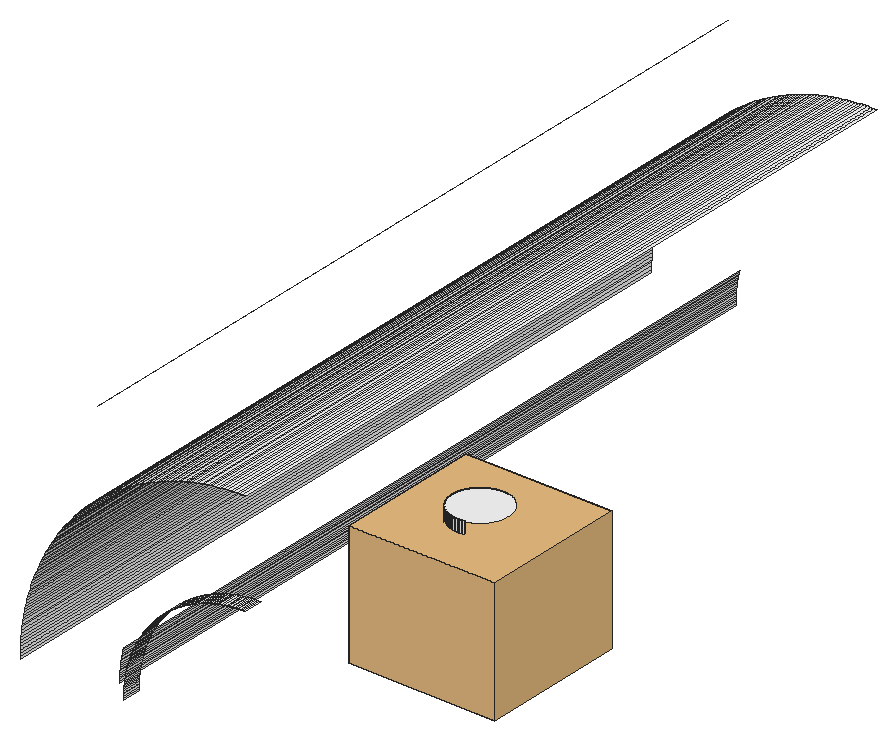
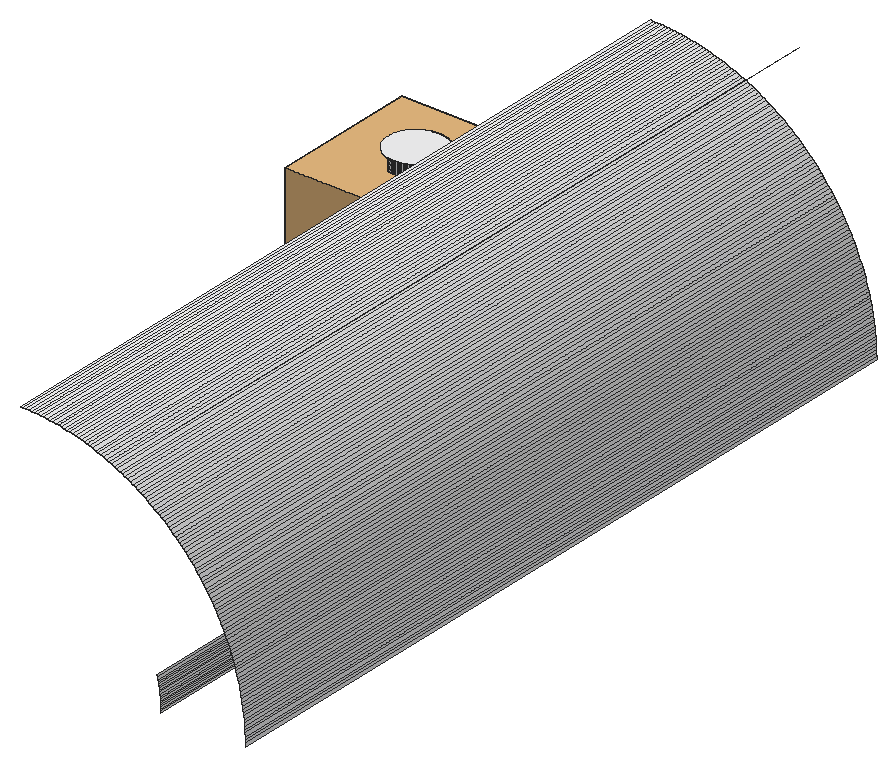
# SketchUp Ruby script. Lengths in inches.
U = 1.inch
M = Sketchup.active_model
def pt(a) = Geom::Point3d.new(a.map { |v| v * U })
def face(e, loops, mat)
  f = e.add_face(loops[0].map { |a| pt(a) })
  loops[1..].each { |l| e.add_face(l.map { |a| pt(a) }).erase! }
  f.material = f.back_material = mat if mat
  f
end
# faces: each face lists its corners as indices into pts; further lists are holes
def faces(e, pts, list, mat = nil) = list.each { |f| face(e, (f[0].is_a?(Array) ? f : [f]).map { |l| l.map { |i| pts[i] } }, mat) }
# xy, xz, yz: faces in a plane at the given z, y or x. An outline is a flat list of corners, or four numbers for a rectangle; further outlines are holes
def ring(l) = l.size == 4 ? [[l[0], l[1]], [l[2], l[1]], [l[2], l[3]], [l[0], l[3]]] : l.each_slice(2).to_a
def flat(e, list, mat, &to3) = list.each { |f| face(e, (f[0].is_a?(Array) ? f : [f]).map { |l| ring(l).map { |u, v| to3.(u, v) } }, mat) }
def xy(e, z, list, mat = nil) = flat(e, list, mat) { |x, y| [x, y, z] }
def xz(e, y, list, mat = nil) = flat(e, list, mat) { |x, z| [x, y, z] }
def yz(e, x, list, mat = nil) = flat(e, list, mat) { |y, z| [x, y, z] }
def lines(e, pts, list) = list.each { |a, b| e.add_line(pt(pts[a]), pt(pts[b])) }
# prism: a flat outline (further loops are holes) pulled along v
def prism(e, loops, v, mat = nil)
  f = face(e, loops, mat); d = Geom::Vector3d.new(v.map { |x| x * U })
  f.pushpull(f.normal.samedirection?(d) ? d.length : -d.length)
end
def box(e, o, s, mat = nil) = prism(e, [[o, [o[0] + s[0], o[1], o[2]], [o[0] + s[0], o[1] + s[1], o[2]], [o[0], o[1] + s[1], o[2]]]], [0, 0, s[2]], mat)
def at(x, y, z, deg = 0) = Geom::Transformation.translation(pt([x, y, z])) * Geom::Transformation.rotation(ORIGIN, Z_AXIS, deg.degrees)
def axes(o, x, y, z) = Geom::Transformation.new([*x, 0, *y, 0, *z, 0, *pt(o).to_a, 1])
def part(name) = M.definitions.add(name)
# library, detail: a bought-in or finely detailed component or shape, given as its bounding box
def library(name, o, s) = part(name).tap { |d| box(d.entities, o, s) }
def detail(e, o, s) = box(e.add_group.entities, o, s)
def put(e, d, t, mat = nil) = e.add_instance(d, t).tap { |i| i.material = mat if mat }
def group(e, t, mat = nil) = e.add_group.tap { |g| g.transformation = t; g.material = mat if mat }.entities
root = M.entities
M.materials.add("[Quartz Light Grey]").color = [251, 251, 252]
c1 = library("5",[-6.25,-6.25,-13.16],[15.58,15.58,13.16])
xy(root,115,[[59.66,187,59.83,189],[59.83,187,60,189]],"[Quartz Light Grey]")
xy(root,119.5,[[68.84,204,68.76,204.01,68.6875,204.02,68.61,204.03,68.45,204.05,68.375,204.07,68.3,204.08,68.22,204.1,68.15,204.125,68.07,204.15,68,204.17,67.92,204.2,67.71,204.29,67.64,204.33,67.57,204.36,67.43,204.44,67.37,204.48,67.3,204.53,67.24,204.57,67.17,204.62,66.93,204.82,66.88,204.88,66.82,204.93,66.62,205.17,66.57,205.24,66.53,205.3,66.48,205.37,66.44,205.43,66.36,205.57,66.33,205.64,66.29,205.71,66.2,205.92,66.17,206,66.15,206.07,66.125,206.15,66.1,206.22,66.08,206.3,66.07,206.375,66.05,206.45,66.03,206.61,66.02,206.6875,66.01,206.76,66,206.84,66,207.16,66.01,207.24,66.02,207.3125,66.03,207.39,66.05,207.55,66.07,207.625,66.08,207.7,66.1,207.78,66.125,207.85,66.15,207.93,66.17,208,66.2,208.08,66.29,208.29,66.33,208.36,66.36,208.43,66.44,208.57,66.48,208.63,66.53,208.7,66.57,208.76,66.62,208.83,66.82,209.07,66.88,209.12,66.93,209.18,67.17,209.38,67.24,209.43,67.3,209.47,67.37,209.52,67.43,209.56,67.57,209.64,67.64,209.67,67.71,209.71,67.92,209.8,68,209.83,68.07,209.85,68.15,209.875,68.22,209.9,68.3,209.92,68.375,209.93,68.45,209.95,68.61,209.97,68.6875,209.98,68.76,209.99,68.84,210,69.16,210,69.24,209.99,69.3125,209.98,69.39,209.97,69.55,209.95,69.625,209.93,69.7,209.92,69.78,209.9,69.85,209.875,69.93,209.85,70,209.83,70.08,209.8,70.29,209.71,70.36,209.67,70.43,209.64,70.57,209.56,70.63,209.52,70.7,209.47,70.76,209.43,70.83,209.38,71.07,209.18,71.12,209.12,71.18,209.07,71.38,208.83,71.43,208.76,71.47,208.7,71.52,208.63,71.56,208.57,71.64,208.43,71.67,208.36,71.71,208.29,71.8,208.08,71.83,208,71.85,207.93,71.875,207.85,71.9,207.78,71.92,207.7,71.93,207.625,71.95,207.55,71.97,207.39,71.98,207.3125,71.99,207.24,72,207.16,72,206.84,71.99,206.76,71.98,206.6875,71.97,206.61,71.95,206.45,71.93,206.375,71.92,206.3,71.9,206.22,71.875,206.15,71.85,206.07,71.83,206,71.8,205.92,71.71,205.71,71.67,205.64,71.64,205.57,71.56,205.43,71.52,205.37,71.47,205.3,71.43,205.24,71.38,205.17,71.18,204.93,71.12,204.88,71.07,204.82,70.83,204.62,70.76,204.57,70.7,204.53,70.63,204.48,70.57,204.44,70.43,204.36,70.36,204.33,70.29,204.29,70.08,204.2,70,204.17,69.93,204.15,69.85,204.125,69.78,204.1,69.7,204.08,69.625,204.07,69.55,204.05,69.39,204.03,69.3125,204.02,69.24,204.01,69.16,204]],"[Quartz Light Grey]")
xy(root,126,[[59.6875,187,60,271]],"[Quartz Light Grey]")
xz(root,204,[[68.84,117,68.92,119.5],[68.92,117,69,119.5],[69,117,69.08,119.5],[69.08,117,69.16,119.5]],"[Quartz Light Grey]")
xz(root,210,[[68.84,117,68.92,119.5],[68.92,117,69,119.5],[69,117,69.08,119.5],[69.08,117,69.16,119.5]],"[Quartz Light Grey]")
yz(root,36,[[187,102,271,102.3125]],"[Quartz Light Grey]")
yz(root,45,[[189,102,271,102.2]],"[Quartz Light Grey]")
yz(root,45.01,[[189,102.39,271,102.59]],"[Quartz Light Grey]")
yz(root,47,[[187,102,189,102.17],[187,102.17,189,102.34]],"[Quartz Light Grey]")
yz(root,66,[[206.84,117,206.92,119.5],[206.92,117,207,119.5],[207,117,207.08,119.5],[207.08,117,207.16,119.5]],"[Quartz Light Grey]")
p = [[45.01,271,102.39],[45.01,189,102.39],[45,189,102.2],[45,271,102.2],[36,187,102.3125],[36.01,187,102.63],
  [36.01,271,102.63],[36,271,102.3125],[47.01,187,102.51],[47,187,102.34],[47,189,102.34],[47.01,189,102.51],
  [47.02,187,102.68],[47.02,189,102.68],[36.02,187,102.94],[36.02,271,102.94],[45.02,271,102.79],[45.02,189,102.79],
  [45.01,189,102.59],[45.01,271,102.59],[47.03,187,102.85],[47.03,189,102.85],[45.03,271,102.98],[45.03,189,102.98],
  [36.03,187,103.26],[36.03,271,103.26],[47.04,187,103.02],[47.04,189,103.02],[47.05,187,103.19],[47.05,189,103.19],
  [45.05,271,103.18],[45.05,189,103.18],[47.07,187,103.36],[47.07,189,103.36],[45.0625,271,103.37],[45.0625,189,103.37],
  [36.05,187,103.57],[36.05,271,103.57],[47.09,187,103.53],[47.09,189,103.53],[45.08,271,103.57],[45.08,189,103.57],
  [47.11,187,103.7],[47.11,189,103.7],[36.07,187,103.88],[36.07,271,103.88],[45.1,271,103.76],[45.1,189,103.76],
  [47.13,187,103.87],[47.13,189,103.87],[45.13,271,103.96],[45.13,189,103.96],[36.1,187,104.2],[36.1,271,104.2],
  [47.16,187,104.03],[47.16,189,104.03],[47.1875,187,104.2],[47.1875,189,104.2],[45.16,271,104.15],[45.16,189,104.15],
  [36.13,187,104.51],[36.13,271,104.51],[47.22,187,104.37],[47.22,189,104.37],[45.18,271,104.35],[45.18,189,104.35],
  [45.22,271,104.54],[45.22,189,104.54],[47.25,187,104.54],[47.25,189,104.54],[36.17,187,104.82],[36.17,271,104.82],
  [47.28,187,104.7],[47.28,189,104.7],[45.25,271,104.73],[45.25,189,104.73],[47.32,187,104.87],[47.32,189,104.87],
  [45.29,271,104.93],[45.29,189,104.93],[36.21,187,105.13],[36.21,271,105.13],[47.36,187,105.03],[47.36,189,105.03],
  [45.33,271,105.12],[45.33,189,105.12],[47.4,187,105.2],[47.4,189,105.2],[36.25,187,105.44],[36.25,271,105.44],
  [45.37,271,105.31],[45.37,189,105.31],[47.44,187,105.36],[47.44,189,105.36],[45.41,271,105.5],[45.41,189,105.5],
  [36.3,187,105.75],[36.3,271,105.75],[47.49,187,105.53],[47.49,189,105.53],[47.54,187,105.69],[47.54,189,105.69],
  [47.58,187,105.86],[47.58,189,105.86],[36.35,187,106.0625],[36.35,271,106.0625],[47.64,187,106.02],[47.64,189,106.02],
  [47.69,187,106.18],[47.69,189,106.18],[36.4,187,106.375],[36.4,271,106.375],[47.75,187,106.34],[47.75,189,106.34],
  [47.8,187,106.5],[47.8,189,106.5],[36.46,187,106.68],[36.46,271,106.68],[47.86,187,106.66],[47.86,189,106.66],
  [36.52,187,106.99],[36.52,271,106.99],[47.93,187,106.82],[47.93,189,106.82],[47.99,187,106.97],[47.99,189,106.97],
  [36.59,187,107.3],[36.59,271,107.3],[48.06,187,107.13],[48.06,189,107.13],[48.125,187,107.29],[48.125,189,107.29],
  [36.66,187,107.6],[36.66,271,107.6],[48.19,187,107.44],[48.19,189,107.44],[48.27,187,107.6],[48.27,189,107.6],
  [36.74,187,107.91],[36.74,271,107.91],[48.34,187,107.75],[48.34,189,107.75],[48.42,187,107.9],[48.42,189,107.9],
  [36.82,187,108.21],[36.82,271,108.21],[48.5,187,108.05],[48.5,189,108.05],[48.58,187,108.2],[48.58,189,108.2],
  [36.9,187,108.51],[36.9,271,108.51],[48.66,187,108.35],[48.66,189,108.35],[48.74,187,108.5],[48.74,189,108.5],
  [36.99,187,108.82],[36.99,271,108.82],[48.83,187,108.65],[48.83,189,108.65],[48.92,187,108.79],[48.92,189,108.79],
  [37.08,187,109.12],[37.08,271,109.12],[49.01,187,108.9375],[49.01,189,108.9375],[49.1,187,109.08],[49.1,189,109.08],
  [37.17,187,109.42],[37.17,271,109.42],[49.19,187,109.22],[49.19,189,109.22],[49.29,187,109.36],[49.29,189,109.36],
  [37.27,187,109.71],[37.27,271,109.71],[49.38,187,109.5],[49.38,189,109.5],[49.48,187,109.64],[49.48,189,109.64],
  [49.58,187,109.78],[49.58,189,109.78],[37.375,187,110.01],[37.375,271,110.01],[49.6875,187,109.91],[49.6875,189,109.91],
  [49.79,187,110.05],[49.79,189,110.05],[37.48,187,110.31],[37.48,271,110.31],[49.9,187,110.18],[49.9,189,110.18],
  [50.01,187,110.3125],[50.01,189,110.3125],[37.59,187,110.6],[37.59,271,110.6],[50.11,187,110.44],[50.11,189,110.44],
  [50.23,187,110.57],[50.23,189,110.57],[37.71,187,110.89],[37.71,271,110.89],[50.34,187,110.7],[50.34,189,110.7],
  [50.45,187,110.82],[50.45,189,110.82],[50.57,187,110.95],[50.57,189,110.95],[37.83,187,111.18],[37.83,271,111.18],
  [50.6875,187,111.07],[50.6875,189,111.07],[50.81,187,111.19],[50.81,189,111.19],[37.95,187,111.47],[37.95,271,111.47],
  [50.93,187,111.3125],[50.93,189,111.3125],[51.05,187,111.43],[51.05,189,111.43],[51.18,187,111.55],[51.18,189,111.55],
  [38.07,187,111.76],[38.07,271,111.76],[51.3,187,111.66],[51.3,189,111.66],[51.43,187,111.77],[51.43,189,111.77],
  [38.2,187,112.05],[38.2,271,112.05],[51.56,187,111.89],[51.56,189,111.89],[51.6875,187,111.99],[51.6875,189,111.99],
  [38.34,187,112.33],[38.34,271,112.33],[51.82,187,112.1],[51.82,189,112.1],[51.95,187,112.21],[51.95,189,112.21],
  [52.09,187,112.3125],[52.09,189,112.3125],[38.48,187,112.61],[38.48,271,112.61],[52.22,187,112.42],[52.22,189,112.42],
  [52.36,187,112.52],[52.36,189,112.52],[52.5,187,112.62],[52.5,189,112.62],[38.62,187,112.9],[38.62,271,112.9],
  [52.64,187,112.71],[52.64,189,112.71],[52.78,187,112.81],[52.78,189,112.81],[52.92,187,112.9],[52.92,189,112.9],
  [38.76,187,113.17],[38.76,271,113.17],[53.0625,187,112.99],[53.0625,189,112.99],[53.21,187,113.08],[53.21,189,113.08],
  [53.35,187,113.17],[53.35,189,113.17],[38.91,187,113.45],[38.91,271,113.45],[53.5,187,113.26],[53.5,189,113.26],
  [53.65,187,113.34],[53.65,189,113.34],[53.8,187,113.42],[53.8,189,113.42],[53.95,187,113.5],[53.95,189,113.5],
  [39.06,187,113.73],[39.06,271,113.73],[54.1,187,113.58],[54.1,189,113.58],[54.25,187,113.66],[54.25,189,113.66],
  [39.22,187,114],[39.22,271,114],[54.4,187,113.73],[54.4,189,113.73],[54.56,187,113.81],[54.56,189,113.81],
  [54.71,187,113.875],[54.71,189,113.875],[54.87,187,113.94],[54.87,189,113.94],[55.03,187,114.01],[55.03,189,114.01],
  [39.375,187,114.27],[39.375,271,114.27],[55.18,187,114.07],[55.18,189,114.07],[55.34,187,114.14],[55.34,189,114.14],
  [55.5,187,114.2],[55.5,189,114.2],[55.66,187,114.25],[55.66,189,114.25],[39.54,187,114.54],[39.54,271,114.54],
  [55.82,187,114.31],[55.82,189,114.31],[55.98,187,114.36],[55.98,189,114.36],[56.14,187,114.42],[56.14,189,114.42],
  [56.31,187,114.46],[56.31,189,114.46],[39.7,187,114.81],[39.7,271,114.81],[56.47,187,114.51],[56.47,189,114.51],
  [56.64,187,114.56],[56.64,189,114.56],[56.8,187,114.6],[56.8,189,114.6],[56.97,187,114.64],[56.97,189,114.64],
  [57.13,187,114.68],[57.13,189,114.68],[57.3,187,114.72],[57.3,189,114.72],[57.46,187,114.75],[57.46,189,114.75],
  [39.87,187,115.07],[39.87,271,115.07],[57.63,187,114.78],[57.63,189,114.78],[57.8,187,114.8125],[57.8,189,114.8125],
  [57.97,187,114.84],[57.97,189,114.84],[58.13,187,114.87],[58.13,189,114.87],[58.3,187,114.89],[58.3,189,114.89],
  [58.47,187,114.91],[58.47,189,114.91],[58.64,187,114.93],[58.64,189,114.93],[58.81,187,114.95],[58.81,189,114.95],
  [58.98,187,114.96],[58.98,189,114.96],[59.15,187,114.97],[59.15,189,114.97],[59.32,187,114.98],[59.32,189,114.98],
  [59.49,187,114.99],[59.49,189,114.99],[59.66,187,115],[59.66,189,115],[40.04,187,115.33],[40.04,271,115.33],
  [40.22,187,115.59],[40.22,271,115.59],[40.4,187,115.85],[40.4,271,115.85],[40.58,187,116.11],[40.58,271,116.11],
  [40.77,187,116.36],[40.77,271,116.36],[40.96,187,116.61],[40.96,271,116.61],[41.15,187,116.86],[41.15,271,116.86],
  [41.35,187,117.1],[41.35,271,117.1],[68.53,204.04,117],[68.45,204.05,117],[68.45,204.05,119.5],[68.53,204.04,119.5],
  [68.61,204.03,117],[68.61,204.03,119.5],[68.6875,204.02,117],[68.6875,204.02,119.5],[68.76,204.01,117],[68.76,204.01,119.5],
  [68.84,204,117],[68.84,204,119.5],[69.24,204.01,117],[69.16,204,117],[69.16,204,119.5],[69.24,204.01,119.5],
  [69.3125,204.02,117],[69.3125,204.02,119.5],[69.39,204.03,117],[69.39,204.03,119.5],[69.47,204.04,117],[69.47,204.04,119.5],
  [69.55,204.05,117],[69.55,204.05,119.5],[68.07,204.15,117],[68,204.17,117],[68,204.17,119.5],[68.07,204.15,119.5],
  [68.15,204.125,117],[68.15,204.125,119.5],[68.22,204.1,117],[68.22,204.1,119.5],[68.3,204.08,117],[68.3,204.08,119.5],
  [68.375,204.07,117],[68.375,204.07,119.5],[69.625,204.07,117],[69.625,204.07,119.5],[69.7,204.08,117],[69.7,204.08,119.5],
  [67.85,204.23,117],[67.78,204.26,117],[67.78,204.26,119.5],[67.85,204.23,119.5],[67.92,204.2,117],[67.92,204.2,119.5],
  [67.64,204.33,117],[67.57,204.36,117],[67.57,204.36,119.5],[67.64,204.33,119.5],[67.71,204.29,117],[67.71,204.29,119.5],
  [67.43,204.44,117],[67.37,204.48,117],[67.37,204.48,119.5],[67.43,204.44,119.5],[67.5,204.4,117],[67.5,204.4,119.5],
  [67.3,204.53,117],[67.24,204.57,117],[67.24,204.57,119.5],[67.3,204.53,119.5],[67.17,204.62,117],[67.11,204.67,117],
  [67.11,204.67,119.5],[67.17,204.62,119.5],[67.05,204.72,117],[66.99,204.77,117],[66.99,204.77,119.5],[67.05,204.72,119.5],
  [66.93,204.82,117],[66.88,204.88,117],[66.88,204.88,119.5],[66.93,204.82,119.5],[66.82,204.93,117],[66.77,204.99,117],
  [66.77,204.99,119.5],[66.82,204.93,119.5],[66.72,205.05,117],[66.72,205.05,119.5],[66.67,205.11,117],[66.62,205.17,117],
  [66.62,205.17,119.5],[66.67,205.11,119.5],[66.57,205.24,117],[66.53,205.3,117],[66.53,205.3,119.5],[66.57,205.24,119.5],
  [66.48,205.37,117],[66.48,205.37,119.5],[66.44,205.43,117],[66.4,205.5,117],[66.4,205.5,119.5],[66.44,205.43,119.5],
  [66.36,205.57,117],[66.36,205.57,119.5],[66.33,205.64,117],[66.29,205.71,117],[66.29,205.71,119.5],[66.33,205.64,119.5],
  [66.26,205.78,117],[66.26,205.78,119.5],[66.23,205.85,117],[66.23,205.85,119.5],[66.2,205.92,117],[66.17,206,117],
  [66.17,206,119.5],[66.2,205.92,119.5],[66.15,206.07,117],[66.15,206.07,119.5],[66.125,206.15,117],[66.1,206.22,117],
  [66.1,206.22,119.5],[66.125,206.15,119.5],[66.08,206.3,117],[66.08,206.3,119.5],[66.07,206.375,117],[66.07,206.375,119.5],
  [66.05,206.45,117],[66.05,206.45,119.5],[66.04,206.53,117],[66.03,206.61,117],[66.03,206.61,119.5],[66.04,206.53,119.5],
  [66.02,206.6875,117],[66.02,206.6875,119.5],[66.01,206.76,117],[66.01,206.76,119.5],[66,206.84,117],[66,206.84,119.5],
  [66,207.16,117],[66.01,207.24,117],[66.01,207.24,119.5],[66,207.16,119.5],[66.02,207.3125,117],[66.02,207.3125,119.5],
  [66.03,207.39,117],[66.03,207.39,119.5],[66.04,207.47,117],[66.04,207.47,119.5],[66.05,207.55,117],[66.05,207.55,119.5],
  [66.07,207.625,117],[66.07,207.625,119.5],[66.08,207.7,117],[66.08,207.7,119.5],[66.1,207.78,117],[66.1,207.78,119.5],
  [66.125,207.85,117],[66.125,207.85,119.5],[66.15,207.93,117],[66.15,207.93,119.5],[66.17,208,117],[66.17,208,119.5],
  [66.2,208.08,117],[66.2,208.08,119.5],[66.23,208.15,117],[66.23,208.15,119.5],[66.26,208.22,117],[66.26,208.22,119.5],
  [66.29,208.29,117],[66.29,208.29,119.5],[66.33,208.36,117],[66.33,208.36,119.5],[66.36,208.43,117],[66.36,208.43,119.5],
  [66.4,208.5,117],[66.4,208.5,119.5],[66.44,208.57,117],[66.44,208.57,119.5],[66.48,208.63,117],[66.48,208.63,119.5],
  [66.53,208.7,117],[66.53,208.7,119.5],[66.57,208.76,117],[66.57,208.76,119.5],[66.62,208.83,117],[66.62,208.83,119.5],
  [66.67,208.89,117],[66.67,208.89,119.5],[66.72,208.95,117],[66.72,208.95,119.5],[66.77,209.01,117],[66.77,209.01,119.5],
  [66.82,209.07,117],[66.82,209.07,119.5],[66.88,209.12,117],[66.88,209.12,119.5],[66.93,209.18,117],[66.93,209.18,119.5],
  [66.99,209.23,117],[66.99,209.23,119.5],[67.05,209.28,117],[67.05,209.28,119.5],[67.11,209.33,117],[67.11,209.33,119.5],
  [67.17,209.38,117],[67.17,209.38,119.5],[67.24,209.43,117],[67.24,209.43,119.5],[67.3,209.47,117],[67.3,209.47,119.5],
  [67.37,209.52,117],[67.37,209.52,119.5],[67.43,209.56,117],[67.43,209.56,119.5],[67.5,209.6,117],[67.5,209.6,119.5],
  [67.57,209.64,117],[67.57,209.64,119.5],[67.64,209.67,117],[67.64,209.67,119.5],[67.71,209.71,117],[67.71,209.71,119.5],
  [67.78,209.74,117],[67.78,209.74,119.5],[67.85,209.77,117],[67.85,209.77,119.5],[67.92,209.8,117],[67.92,209.8,119.5],
  [68,209.83,117],[68,209.83,119.5],[68.07,209.85,117],[68.07,209.85,119.5],[68.15,209.875,117],[68.15,209.875,119.5],
  [68.22,209.9,117],[68.22,209.9,119.5],[68.3,209.92,117],[68.3,209.92,119.5],[68.375,209.93,117],[68.375,209.93,119.5],
  [68.45,209.95,117],[68.45,209.95,119.5],[68.53,209.96,117],[68.53,209.96,119.5],[69.47,209.96,117],[69.55,209.95,117],
  [69.55,209.95,119.5],[69.47,209.96,119.5],[69.625,209.93,117],[69.625,209.93,119.5],[69.7,209.92,117],[69.7,209.92,119.5],
  [68.61,209.97,117],[68.61,209.97,119.5],[68.6875,209.98,117],[68.6875,209.98,119.5],[68.76,209.99,117],[68.76,209.99,119.5],
  [68.84,210,117],[68.84,210,119.5],[69.16,210,117],[69.24,209.99,117],[69.24,209.99,119.5],[69.16,210,119.5],
  [69.3125,209.98,117],[69.3125,209.98,119.5],[69.39,209.97,117],[69.39,209.97,119.5],[41.55,187,117.35],[41.55,271,117.35],
  [41.75,187,117.59],[41.75,271,117.59],[41.96,187,117.82],[41.96,271,117.82],[42.16,187,118.06],[42.16,271,118.06],
  [42.375,187,118.29],[42.375,271,118.29],[42.59,187,118.52],[42.59,271,118.52],[42.81,187,118.75],[42.81,271,118.75],
  [43.03,187,118.97],[43.03,271,118.97],[43.25,187,119.19],[43.25,271,119.19],[43.48,187,119.41],[43.48,271,119.41],
  [43.71,187,119.625],[43.71,271,119.625],[43.94,187,119.84],[43.94,271,119.84],[44.18,187,120.04],[44.18,271,120.04],
  [44.41,187,120.25],[44.41,271,120.25],[44.65,187,120.45],[44.65,271,120.45],[44.9,187,120.65],[44.9,271,120.65],
  [45.14,187,120.85],[45.14,271,120.85],[45.39,187,121.04],[45.39,271,121.04],[45.64,187,121.23],[45.64,271,121.23],
  [45.89,187,121.42],[45.89,271,121.42],[46.15,187,121.6],[46.15,271,121.6],[46.41,187,121.78],[46.41,271,121.78],
  [46.67,187,121.96],[46.67,271,121.96],[46.93,187,122.13],[46.93,271,122.13],[47.19,187,122.3],[47.19,271,122.3],
  [47.46,187,122.46],[47.46,271,122.46],[47.73,187,122.625],[47.73,271,122.625],[48,187,122.78],[48,271,122.78],
  [48.27,187,122.94],[48.27,271,122.94],[48.55,187,123.09],[48.55,271,123.09],[48.83,187,123.24],[48.83,271,123.24],
  [49.1,187,123.38],[49.1,271,123.38],[49.39,187,123.52],[49.39,271,123.52],[49.67,187,123.66],[49.67,271,123.66],
  [49.95,187,123.8],[49.95,271,123.8],[50.24,187,123.93],[50.24,271,123.93],[50.53,187,124.05],[50.53,271,124.05],
  [50.82,187,124.17],[50.82,271,124.17],[51.11,187,124.29],[51.11,271,124.29],[51.4,187,124.41],[51.4,271,124.41],
  [51.69,187,124.52],[51.69,271,124.52],[51.99,187,124.625],[51.99,271,124.625],[52.29,187,124.73],[52.29,271,124.73],
  [52.58,187,124.83],[52.58,271,124.83],[52.88,187,124.92],[52.88,271,124.92],[53.18,187,125.01],[53.18,271,125.01],
  [53.49,187,125.1],[53.49,271,125.1],[53.79,187,125.18],[53.79,271,125.18],[54.09,187,125.26],[54.09,271,125.26],
  [54.4,187,125.34],[54.4,271,125.34],[54.7,187,125.41],[54.7,271,125.41],[55.01,187,125.48],[55.01,271,125.48],
  [55.32,187,125.54],[55.32,271,125.54],[55.625,187,125.6],[55.625,271,125.6],[55.9375,187,125.65],[55.9375,271,125.65],
  [56.25,187,125.7],[56.25,271,125.7],[56.56,187,125.75],[56.56,271,125.75],[56.87,187,125.79],[56.87,271,125.79],
  [57.18,187,125.83],[57.18,271,125.83],[57.49,187,125.87],[57.49,271,125.87],[57.8,187,125.9],[57.8,271,125.9],
  [58.12,187,125.93],[58.12,271,125.93],[58.43,187,125.95],[58.43,271,125.95],[58.74,187,125.97],[58.74,271,125.97],
  [59.06,187,125.98],[59.06,271,125.98],[59.37,187,125.99],[59.37,271,125.99],[59.6875,187,126],[59.6875,271,126],
  [44.18,271,128.99],[44.18,187,128.99]]
faces(root,p,[[0,1,2,3],[4,5,6,7],[8,9,10,11],[12,8,11,13],[5,14,15,6],[16,17,18,19],[20,12,13,21],[22,23,17,16],
  [14,24,25,15],[26,20,21,27],[28,26,27,29],[30,31,23,22],[32,28,29,33],[34,35,31,30],[24,36,37,25],[38,32,33,39],
  [40,41,35,34],[42,38,39,43],[36,44,45,37],[46,47,41,40],[48,42,43,49],[50,51,47,46],[44,52,53,45],[54,48,49,55],
  [56,54,55,57],[58,59,51,50],[52,60,61,53],[62,56,57,63],[64,65,59,58],[66,67,65,64],[68,62,63,69],[60,70,71,61],
  [72,68,69,73],[74,75,67,66],[76,72,73,77],[78,79,75,74],[70,80,81,71],[82,76,77,83],[84,85,79,78],[86,82,83,87],
  [80,88,89,81],[90,91,85,84],[92,86,87,93],[94,95,91,90],[88,96,97,89],[98,92,93,99],[100,98,99,101],[102,100,101,103],
  [96,104,105,97],[106,102,103,107],[108,106,107,109],[104,110,111,105],[112,108,109,113],[114,112,113,115],[110,116,117,111],[118,114,115,119],
  [116,120,121,117],[122,118,119,123],[124,122,123,125],[120,126,127,121],[128,124,125,129],[130,128,129,131],[126,132,133,127],[134,130,131,135],
  [136,134,135,137],[132,138,139,133],[140,136,137,141],[142,140,141,143],[138,144,145,139],[146,142,143,147],[148,146,147,149],[144,150,151,145],
  [152,148,149,153],[154,152,153,155],[150,156,157,151],[158,154,155,159],[160,158,159,161],[156,162,163,157],[164,160,161,165],[166,164,165,167],
  [162,168,169,163],[170,166,167,171],[172,170,171,173],[168,174,175,169],[176,172,173,177],[178,176,177,179],[180,178,179,181],[174,182,183,175],
  [184,180,181,185],[186,184,185,187],[182,188,189,183],[190,186,187,191],[192,190,191,193],[188,194,195,189],[196,192,193,197],[198,196,197,199],
  [194,200,201,195],[202,198,199,203],[204,202,203,205],[206,204,205,207],[200,208,209,201],[210,206,207,211],[212,210,211,213],[208,214,215,209],
  [216,212,213,217],[218,216,217,219],[220,218,219,221],[214,222,223,215],[224,220,221,225],[226,224,225,227],[222,228,229,223],[230,226,227,231],
  [232,230,231,233],[228,234,235,229],[236,232,233,237],[238,236,237,239],[240,238,239,241],[234,242,243,235],[244,240,241,245],[246,244,245,247],
  [248,246,247,249],[242,250,251,243],[252,248,249,253],[254,252,253,255],[256,254,255,257],[250,258,259,251],[260,256,257,261],[262,260,261,263],
  [264,262,263,265],[258,266,267,259],[268,264,265,269],[270,268,269,271],[272,270,271,273],[274,272,273,275],[266,276,277,267],[278,274,275,279],
  [280,278,279,281],[276,282,283,277],[284,280,281,285],[286,284,285,287],[288,286,287,289],[290,288,289,291],[292,290,291,293],[282,294,295,283],
  [296,292,293,297],[298,296,297,299],[300,298,299,301],[302,300,301,303],[294,304,305,295],[306,302,303,307],[308,306,307,309],[310,308,309,311],
  [312,310,311,313],[304,314,315,305],[316,312,313,317],[318,316,317,319],[320,318,319,321],[322,320,321,323],[324,322,323,325],[326,324,325,327],
  [328,326,327,329],[314,330,331,315],[332,328,329,333],[334,332,333,335],[336,334,335,337],[338,336,337,339],[340,338,339,341],[342,340,341,343],
  [344,342,343,345],[346,344,345,347],[348,346,347,349],[350,348,349,351],[352,350,351,353],[354,352,353,355],[356,354,355,357],[330,358,359,331],
  [358,360,361,359],[360,362,363,361],[362,364,365,363],[364,366,367,365],[366,368,369,367],[368,370,371,369],[370,372,373,371],[374,375,376,377],
  [378,374,377,379],[380,378,379,381],[382,380,381,383],[384,382,383,385],[386,387,388,389],[390,386,389,391],[392,390,391,393],[394,392,393,395],
  [396,394,395,397],[398,399,400,401],[402,398,401,403],[404,402,403,405],[406,404,405,407],[408,406,407,409],[375,408,409,376],[410,396,397,411],
  [412,410,411,413],[414,415,416,417],[418,414,417,419],[399,418,419,400],[420,421,422,423],[424,420,423,425],[415,424,425,416],[426,427,428,429],
  [430,426,429,431],[421,430,431,422],[432,433,434,435],[427,432,435,428],[436,437,438,439],[433,436,439,434],[440,441,442,443],[437,440,443,438],
  [444,445,446,447],[441,444,447,442],[448,449,450,451],[445,448,451,446],[449,452,453,450],[454,455,456,457],[452,454,457,453],[458,459,460,461],
  [455,458,461,456],[459,462,463,460],[464,465,466,467],[462,464,467,463],[465,468,469,466],[470,471,472,473],[468,470,473,469],[471,474,475,472],
  [474,476,477,475],[478,479,480,481],[476,478,481,477],[479,482,483,480],[484,485,486,487],[482,484,487,483],[485,488,489,486],[488,490,491,489],
  [490,492,493,491],[494,495,496,497],[492,494,497,493],[495,498,499,496],[498,500,501,499],[500,502,503,501],[504,505,506,507],[505,508,509,506],
  [508,510,511,509],[510,512,513,511],[512,514,515,513],[514,516,517,515],[516,518,519,517],[518,520,521,519],[520,522,523,521],[522,524,525,523],
  [524,526,527,525],[526,528,529,527],[528,530,531,529],[530,532,533,531],[532,534,535,533],[534,536,537,535],[536,538,539,537],[538,540,541,539],
  [540,542,543,541],[542,544,545,543],[544,546,547,545],[546,548,549,547],[548,550,551,549],[550,552,553,551],[552,554,555,553],[554,556,557,555],
  [556,558,559,557],[558,560,561,559],[560,562,563,561],[562,564,565,563],[564,566,567,565],[566,568,569,567],[568,570,571,569],[570,572,573,571],
  [572,574,575,573],[574,576,577,575],[576,578,579,577],[578,580,581,579],[580,582,583,581],[582,584,585,583],[584,586,587,585],[586,588,589,587],
  [588,590,591,589],[590,592,593,591],[592,594,595,593],[594,596,597,595],[596,598,599,597],[598,600,601,599],[600,602,603,601],[602,604,605,603],
  [604,606,607,605],[606,608,609,607],[610,611,612,613],[611,614,615,612],[614,616,617,615],[608,618,619,609],[618,620,621,619],[620,622,623,621],
  [622,624,625,623],[626,627,628,629],[627,630,631,628],[630,632,633,631],[632,610,613,633],[372,634,635,373],[634,636,637,635],[636,638,639,637],
  [638,640,641,639],[640,642,643,641],[642,644,645,643],[644,646,647,645],[646,648,649,647],[648,650,651,649],[650,652,653,651],[652,654,655,653],
  [654,656,657,655],[656,658,659,657],[658,660,661,659],[660,662,663,661],[662,664,665,663],[664,666,667,665],[666,668,669,667],[668,670,671,669],
  [670,672,673,671],[672,674,675,673],[674,676,677,675],[676,678,679,677],[678,680,681,679],[680,682,683,681],[682,684,685,683],[684,686,687,685],
  [686,688,689,687],[688,690,691,689],[690,692,693,691],[692,694,695,693],[694,696,697,695],[696,698,699,697],[698,700,701,699],[700,702,703,701],
  [702,704,705,703],[704,706,707,705],[706,708,709,707],[708,710,711,709],[710,712,713,711],[712,714,715,713],[714,716,717,715],[716,718,719,717],
  [718,720,721,719],[720,722,723,721],[722,724,725,723],[724,726,727,725],[726,728,729,727],[728,730,731,729],[730,732,733,731],[732,734,735,733],
  [734,736,737,735],[736,738,739,737],[738,740,741,739],[740,742,743,741],[742,744,745,743],[744,746,747,745],[746,748,749,747],[748,750,751,749],
  [750,752,753,751],[752,754,755,753],[754,756,757,755],[756,758,759,757],[758,760,761,759],[760,762,763,761],[762,764,765,763],[764,766,767,765]],"[Quartz Light Grey]")
lines(root,p,[[768,769]])
put(root,c1,at(67.46,205.47,118.25),"[Quartz Light Grey]")
